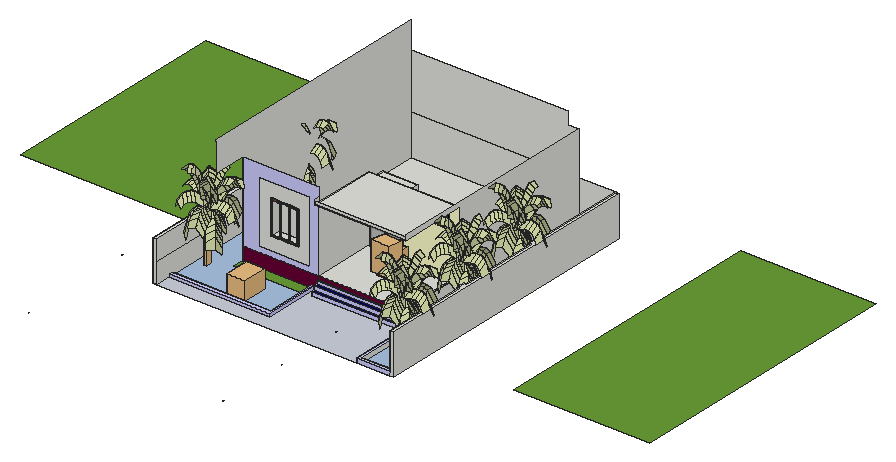
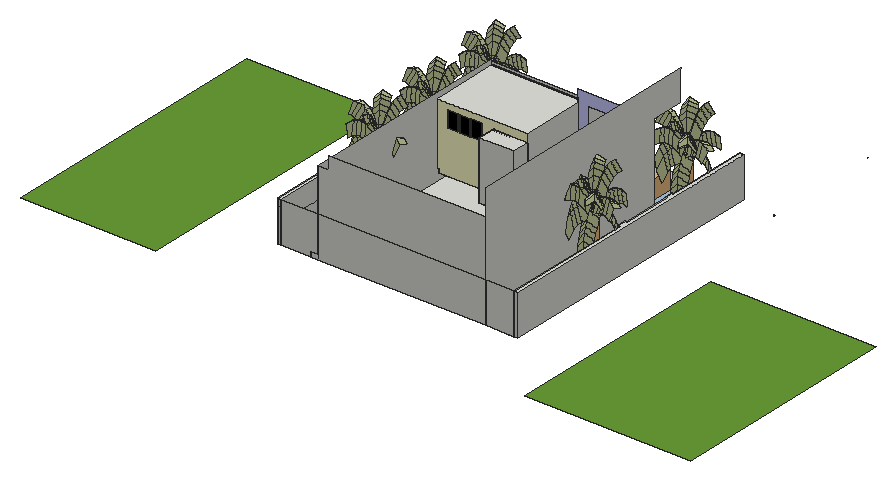
# SketchUp Ruby script. Lengths in inches.
U = 1.inch
M = Sketchup.active_model
def pt(a) = Geom::Point3d.new(a.map { |v| v * U })
def face(e, loops, mat)
  f = e.add_face(loops[0].map { |a| pt(a) })
  loops[1..].each { |l| e.add_face(l.map { |a| pt(a) }).erase! }
  f.material = f.back_material = mat if mat
  f
end
# faces: each face lists its corners as indices into pts; further lists are holes
def faces(e, pts, list, mat = nil) = list.each { |f| face(e, (f[0].is_a?(Array) ? f : [f]).map { |l| l.map { |i| pts[i] } }, mat) }
# xy, xz, yz: faces in a plane at the given z, y or x. An outline is a flat list of corners, or four numbers for a rectangle; further outlines are holes
def ring(l) = l.size == 4 ? [[l[0], l[1]], [l[2], l[1]], [l[2], l[3]], [l[0], l[3]]] : l.each_slice(2).to_a
def flat(e, list, mat, &to3) = list.each { |f| face(e, (f[0].is_a?(Array) ? f : [f]).map { |l| ring(l).map { |u, v| to3.(u, v) } }, mat) }
def xy(e, z, list, mat = nil) = flat(e, list, mat) { |x, y| [x, y, z] }
def xz(e, y, list, mat = nil) = flat(e, list, mat) { |x, z| [x, y, z] }
def yz(e, x, list, mat = nil) = flat(e, list, mat) { |y, z| [x, y, z] }
def lines(e, pts, list) = list.each { |a, b| e.add_line(pt(pts[a]), pt(pts[b])) }
# prism: a flat outline (further loops are holes) pulled along v
def prism(e, loops, v, mat = nil)
  f = face(e, loops, mat); d = Geom::Vector3d.new(v.map { |x| x * U })
  f.pushpull(f.normal.samedirection?(d) ? d.length : -d.length)
end
def box(e, o, s, mat = nil) = prism(e, [[o, [o[0] + s[0], o[1], o[2]], [o[0] + s[0], o[1] + s[1], o[2]], [o[0], o[1] + s[1], o[2]]]], [0, 0, s[2]], mat)
def at(x, y, z, deg = 0) = Geom::Transformation.translation(pt([x, y, z])) * Geom::Transformation.rotation(ORIGIN, Z_AXIS, deg.degrees)
def axes(o, x, y, z) = Geom::Transformation.new([*x, 0, *y, 0, *z, 0, *pt(o).to_a, 1])
def part(name) = M.definitions.add(name)
# library, detail: a bought-in or finely detailed component or shape, given as its bounding box
def library(name, o, s) = part(name).tap { |d| box(d.entities, o, s) }
def detail(e, o, s) = box(e.add_group.entities, o, s)
def put(e, d, t, mat = nil) = e.add_instance(d, t).tap { |i| i.material = mat if mat }
def group(e, t, mat = nil) = e.add_group.tap { |g| g.transformation = t; g.material = mat if mat }.entities
root = M.entities
M.materials.add("Wall-Decor-Art-Painting-YH-W-005-").color = [116, 59, 36]
M.materials.add("Wall-Decor-Art-Painting-YH-W-005- copy").color = [132, 50, 31]
M.materials.add("Wall-Decor-Art-Painting-YH-W-005- copy 2").color = [130, 72, 41]
M.materials.add("Wine2").color = [0, 0, 0]
M.materials["Wine2"].alpha = 0
M.materials.add("[0130_Gainsboro]").color = [39, 45, 50]
M.materials.add("[Color E01]").color = [255, 255, 204]
M.materials.add("[Color I01]").color = [204, 204, 255]
M.materials.add("[Color I08]").color = [0, 0, 102]
M.materials.add("[Color L16]").color = [102, 0, 51]
M.materials.add("[Color M00]").color = [255, 255, 255]
M.materials.add("[Color_002]").color = [198, 198, 198]
M.materials.add("[Color_009]").color = [0, 0, 0]
M.materials.add("[Grass Dark Green]").color = [106, 157, 55]
M.materials.add("[Marble Carrara Floor Tile]").color = [204, 208, 219]
M.materials.add("[Mosaic Hexagonal Tile]").color = [168, 194, 223]
M.materials.add("[Translucent_Resin_Crush_Gray]").color = [184, 184, 184]
M.materials["[Translucent_Resin_Crush_Gray]"].alpha = 0.8
M.materials.add("[Wood Floor Parquet]").color = [145, 89, 39]
M.materials.add("[Wood_Cherry_Original]").color = [152, 86, 42]
M.materials.add("leaf").color = [206, 213, 162]
M.materials.add("top").color = [180, 165, 147]
M.materials.add("Рамы 2").color = [204, 204, 204]
c1 = library("water+(1)",[16,-149.35,-6.82],[116.59,156.63,119.32])
c2 = library("Palm trunk",[157.4375,124.31,0],[15.93,35.48,172.86])
c3 = part("Group\#7")
p = [[164.1,0,77.84],[148.54,0,92.1],[148.54,41.93,119.66],[173.71,41.93,96.59],[148.54,83.86,92.1],[164.1,83.86,77.84],
  [5.38,41.93,118.9],[46.17,41.93,129.83],[46.17,0,102.27],[5.38,0,91.34],[5.38,83.86,91.34],[46.17,83.86,102.27],
  [129.8125,41.93,129.41],[129.8125,0,101.85],[129.8125,83.86,101.85],[109.2,41.93,133.98],[109.2,0,106.42],[109.2,83.86,106.42],
  [88.1,41.93,134.75],[88.1,0,107.19],[88.1,83.86,107.19]]
faces(c3.entities,p,[[0,1,2,3],[3,2,4,5],[6,7,8,9],[10,11,7,6],[12,2,1,13],[14,4,2,12],[15,12,13,16],[17,14,12,15],
  [7,18,19,8],[11,20,18,7],[18,15,16,19],[20,17,15,18]],"leaf")
c4 = part("Coconut palm")
put(c4.entities,c2,at(0,-1.57,0))
put(c4.entities,c3,axes([81.77,133.63,84.54],[0.69255,-0.55067,-0.46599],[0.5,0.83206,-0.24016],[0.51998,-0.06667,0.85157]))
g1 = group(c4.entities,at(162.91,84.37,70.6))
p = [[173.91,67.02,81],[148.54,73.47,103.34],[148.54,106.11,65.23],[164.1,102.16,51.53],[5.38,105.9,64.5],[46.17,108.93,75],
  [46.17,76.29,113.11],[5.38,73.26,102.61],[129.8125,108.8125,74.6],[129.8125,76.17,112.71],[109.2,110.08,78.99],[109.2,77.4375,117.1],
  [164.1,21.59,74.79],[148.54,25.54,88.49],[88.1,110.3,79.73],[88.1,77.65,117.84],[46.17,28.36,98.26],[5.38,25.33,87.76],
  [129.8125,28.24,97.86],[109.2,29.51,102.25],[88.1,29.73,102.99]]
faces(g1,p,[[0,1,2,3],[4,5,6,7],[8,2,1,9],[10,8,9,11],[12,13,1,0],[5,14,15,6],[14,10,11,15],[7,6,16,17],
  [9,1,13,18],[11,9,18,19],[6,15,20,16],[15,11,19,20]],"leaf")
g2 = group(c4.entities,at(165.48,195.56,135.875))
p = [[-108.28,-70.71,-19.53],[-87.32,-105.59,-9.46],[-94.61,-121.11,-48.04],[-115.57,-86.22,-58.11],[-60.61,-153.8125,-57.55],[-53.31,-138.3,-18.96],
  [-98.87,-60.46,-3.65],[-77.9,-95.35,6.42],[-43.9,-128.05,-3.08],[-64.02,-83.84,17.4],[-84.98,-48.95,7.33],[-30.02,-116.54,7.9],
  [-32.71,-60.42,33.34],[-53.67,-25.54,23.27],[1.3,-93.125,23.84],[-18.16,-3.04,27.26],[2.8,-37.93,37.33],[36.81,-70.63,27.83]]
faces(g2,p,[[0,1,2,3],[4,2,1,5],[6,7,1,0],[8,5,1,7],[9,7,6,10],[11,8,7,9],[12,9,10,13],[14,11,9,12],
  [15,16,12,13],[14,12,16,17]],"leaf")
g3 = group(c4.entities,at(142.62,171.34,50.42))
p = [[25.67,-13.71,122.79],[-8.79,-1.2,143.75],[-10.19,32.74,106.83],[24.26,20.24,85.87],[-46.23,10.35,159.48],[-47.64,44.3,122.56],
  [9.41,-59.05,108.76],[-25.04,-46.55,129.72],[-127.77,57.3125,115.67],[-108.71,56.35,124.71],[-107.31,22.41,161.625],[-138.46,23.97,146.85],
  [-66.11,15.49,164.38],[-67.52,49.44,127.46],[-86.76,19.72,165.65],[-88.16,53.67,128.73],[-62.49,-35,145.45],[-123.5625,-22.94,147.59],
  [-142.62,-21.98,138.55],[-82.37,-29.86,150.35],[-103.01,-25.63,151.62]]
faces(g3,p,[[0,1,2,3],[1,4,5,2],[6,7,1,0],[8,9,10,11],[4,12,13,5],[14,10,9,15],[12,14,15,13],[7,16,4,1],
  [11,10,17,18],[16,19,12,4],[20,17,10,14],[19,20,14,12]],"leaf")
g4 = group(c4.entities,at(218.66,104.39,70.49))
p = [[-50.44,173.74,-16.1],[-47.24,168.22,4.03],[-89.48,170.8,30.99],[-95.125,180.54,-4.51],[-127.6875,145.47,10.59],[-130.89,150.99,-9.53],
  [-85.08,160.41,48.83],[-42.84,157.83,21.87],[-123.29,135.08,28.4375],[-79.79,145.86,63.18],[-37.56,143.27,36.22],[-118,120.53,42.79],
  [-74.1,128.98,74.51],[-31.86,126.4,47.55],[-112.31,103.65,54.12],[-62.3,92.16,91.49],[-20.0625,89.58,64.52],[-100.51,66.83,71.09],
  [-50.38,53.24,102.72],[-8.14,50.66,75.76],[-88.59,27.91,82.32]]
faces(g4,p,[[0,1,2,3],[3,2,4,5],[6,2,1,7],[8,4,2,6],[9,6,7,10],[11,8,6,9],[12,9,10,13],[14,11,9,12],
  [15,12,13,16],[17,14,12,15],[18,15,16,19],[20,17,15,18]],"leaf")
g5 = group(c4.entities,at(210.73,128.28,159.9))
p = [[6.68,160.75,-68.99],[43.02,158.53,-41.125],[14.09,136.62,-0.32],[-15.69,143.8,-37.44],[49.16,120.18,15.72],[71.53,137.12,-15.83],
  [-27.22,129.99,-26.4],[2.56,122.8,10.72],[-37.86,112.57,-21],[-8.08,105.38,16.11],[-57.34,75.37,-16.54],[-27.56,68.1875,20.58],
  [-42.45,29.35,13.31],[-72.23,36.53,-23.81],[37.63,106.36,26.76],[27,88.9375,32.16],[-7.375,12.9,29.35],[7.51,51.74,36.62]]
faces(g5,p,[[0,1,2,3],[4,2,1,5],[6,3,2,7],[8,6,7,9],[10,11,12,13],[10,8,9,11],[14,7,2,4],[9,7,14,15],
  [16,12,11,17],[11,9,15,17]],"leaf")
g6 = group(c4.entities,at(98.15,94.13,89.7))
p = [[70.13,63.5,83.51],[57.26,51.26,121.8125],[12.59,51.35,98.97],[25.46,63.59,60.66],[98.15,23.43,72.25],[85.28,11.19,110.5625],
  [42.12,34.09,157.3],[-2.55,34.18,134.45],[70.14,-5.98,146.04],[33.52,23.1,173.14],[-11.15,23.19,150.29],[61.54,-16.97,161.88],
  [23.97,9.59,186.25],[-20.71,9.68,163.41],[51.99,-30.48,175],[13.59,-6.74,194.7],[-31.08,-6.65,171.86],[-41.56,-24.69,175.08],
  [3.11,-24.78,197.92],[41.62,-46.8125,183.45],[31.14,-64.85,186.67]]
faces(g6,p,[[0,1,2,3],[4,5,1,0],[1,6,7,2],[5,8,6,1],[6,9,10,7],[8,11,9,6],[9,12,13,10],[11,14,12,9],
  [12,15,16,13],[17,16,15,18],[14,19,15,12],[18,15,19,20]],"leaf")
g7 = group(c4.entities,at(200.43,222.47,102.78))
p = [[-53.13,-46.15,54.03],[-52.26,-28.65,85.38],[-31.27,-47.33,101.78],[-32.14,-64.84,70.43],[-6,-33.4,86.75],[-6.87,-50.9,55.4],
  [-50.88,-6.91,114.01],[-29.89,-25.6,130.42],[-4.62,-11.66,115.38],[-49.93,5.95,126.57],[-28.94,-12.74,142.97],[-3.67,1.2,127.9375],
  [-48.71,20.77,136.65],[-27.72,2.08,153.05],[-2.45,16.02,138.02],[-47.16,37.54,142.625],[-26.17,18.86,159.03],[-0.9,32.79,144],
  [-23.3125,47.39,161.38],[-45.4,55.14,144.08],[0.86,50.39,145.45]]
faces(g7,p,[[0,1,2,3],[3,2,4,5],[1,6,7,2],[2,7,8,4],[6,9,10,7],[7,10,11,8],[9,12,13,10],[10,13,14,11],
  [12,15,16,13],[13,16,17,14],[18,16,15,19],[20,17,16,18]],"leaf")
g8 = group(c4.entities,at(245.82,148.18,74.1))
p = [[-95.45,43.17,66.56],[-77.22,70.01,93.58],[-59.3125,36.28,126.13],[-77.54,9.45,99.11],[-17.82,13.13,110],[-36.05,-13.7,82.97],
  [-55.78,98.8125,115.8],[-37.87,65.09,148.35],[3.62,41.9375,132.21],[-43.61,113.93,124.1],[-25.69,80.2,156.65],[26.92,133.51,150.95],
  [2.52,110.86,160.76],[-15.39,144.58,128.21],[-0.55,158.36,122.24],[-30.08,129.43,128.85],[-12.17,95.7,161.4],[15.79,57.05,140.52],
  [58.85,101.49,138.66],[44.01,87.71,144.625],[29.32,72.55,145.26]]
faces(g8,p,[[0,1,2,3],[3,2,4,5],[1,6,7,2],[2,7,8,4],[6,9,10,7],[11,12,13,14],[9,15,16,10],[15,13,12,16],
  [7,10,17,8],[18,19,12,11],[10,16,20,17],[16,12,19,20]],"leaf")
g9 = group(c4.entities,at(184.07,231.3125,71.99))
p = [[-52.97,-87.38,70.44],[-75.91,-65.15,98.06],[-38.73,-51.45,128.83],[-15.79,-73.68,101.22],[-10.82,-13.84,110.82],[12.12,-36.07,83.21],
  [-100.5625,-39.55,120.86],[-63.375,-25.85,151.64],[-35.47,11.76,133.625],[-113.51,-25.26,129.46],[-76.32,-11.57,160.23],[-122.54,48.32,155.17],
  [-102.64,20.66,164.86],[-139.82,6.97,134.09],[-151.68,23.45,128.31],[-126.8,-9.65,134.48],[-89.62,4.05,165.25],[-48.42,26.05,142.22],
  [-86.59,74.76,141.07],[-74.73,58.28,146.85],[-61.71,41.66,147.24]]
faces(g9,p,[[0,1,2,3],[3,2,4,5],[1,6,7,2],[2,7,8,4],[6,9,10,7],[11,12,13,14],[9,15,16,10],[7,10,17,8],
  [15,13,12,16],[18,19,12,11],[10,16,20,17],[16,12,19,20]],"leaf")
g10 = group(c4.entities,at(155.33,63.22,90.49))
p = [[56.62,93.99,58],[69.99,76.62,94.09],[26.33,77.04,118.8125],[12.96,94.41,82.72],[-4.99,40.54,104.5],[-18.36,57.91,68.41],
  [85.15,54.53,126.73],[41.49,54.95,151.45],[10.16,18.46,137.14],[93.5,41.24,140.85],[49.84,41.66,165.57],[18.52,5.17,151.26],
  [102.52,25.71,151.94],[58.86,26.125,176.66],[27.53,-10.37,162.35],[111.96,7.84,158.06],[68.3,8.26,182.78],[83.97,-23.96,184],
  [121.19,-11.13,158.78],[36.98,-28.23,168.47],[46.21,-47.21,169.1875]]
faces(g10,p,[[0,1,2,3],[3,2,4,5],[1,6,7,2],[2,7,8,4],[6,9,10,7],[7,10,11,8],[9,12,13,10],[10,13,14,11],
  [12,15,16,13],[17,16,15,18],[13,16,19,14],[20,19,16,17]],"leaf")
g11 = group(c4.entities,at(143.97,131.21,156.06))
p = [[28.02,18.96,27.99],[28.02,5.02,30.3],[22.98,-0.55,-3.35],[22.98,16.04,-6.1],[22.98,22.36,-7.14],[22.98,28.6875,-8.1875],
  [22.98,45.28,-10.9375],[28.02,50.85,22.71],[28.02,36.91,25.02],[28.02,27.9375,26.51],[37.15,27.72,25.18],[51,27.38,23.16],
  [45.96,21.8125,-10.49],[29.41,22.21,-8.08],[16.55,22.52,-6.21],[0,22.92,-3.79],[5.04,28.49,29.86],[18.89,28.16,27.84],
  [29.9,23.86,-8.43],[25,29.125,-8.5625],[30.88,37.53,24.49],[34.36,33.8,24.59],[37.84,30.06,24.6875],[18.08,27.63,-7.28],
  [21.06,35.41,26.3125],[27.89,17.1,-7.01],[34.98,20.46,26.7],[16.0625,20.87,-5.86],[18.19,25.8125,28.33],[25.16,18.34,28.53],
  [20.97,15.61,-5.72],[21.67,22.07,28.43]]
faces(g11,p,[[0,1,2,3,4,5,6,7,8,9],[10,11,12,13,4,14,15,16,17,9],[18,19,20,21,22],[23,24,8,20,19,5],[25,13,18,22,10,26],[17,24,23,14,27,28],[25,26,0,29,30,3],[31,28,27,30,29]],"top")
g12 = group(c4.entities,at(232.25,84.82,92.39))
p = [[-43.76,105.5,48.57],[-18.03,112.66,81.27],[-38.24,79.96,113.53],[-63.96,72.8,80.82],[-25.16,32.38,104.44],[-50.89,25.22,71.74],
  [12.23,118.3125,110.17],[-7.97,85.62,142.42],[5.11,38.03,133.34],[29.42,120.28,122.27],[9.22,87.58,154.52],[48.52,121.17,131.23],
  [28.3125,88.47,163.48],[69.25,120.47,135.17],[49.04,87.77,167.43],[22.3,40,145.4375],[84.11,84.01,165.18],[90.19,118.22,133.83],
  [41.39,40.89,154.4],[62.12,40.1875,158.34],[83.07,37.94,157]]
faces(g12,p,[[0,1,2,3],[3,2,4,5],[1,6,7,2],[2,7,8,4],[6,9,10,7],[9,11,12,10],[11,13,14,12],[7,10,15,8],
  [16,14,13,17],[10,12,18,15],[12,14,19,18],[20,19,14,16]],"leaf")
g13 = group(c4.entities,at(137.93,152.93,50.82))
p = [[30.35,4.7,122.39],[5.92,-23.64,141.95],[-27.65,-7.16,108.51],[-3.22,21.19,88.95],[63.93,-27.07,102.88],[39.49,-55.42,122.4375],
  [-19.2,-54.54,156],[-52.77,-38.05,122.55],[-98.3,-104.66,111.23],[-88.98,-88.73,121.47],[-55.4,-105.22,154.92],[-70.46,-130.95,138.37],
  [-44.1875,-88.11,160.125],[-77.76,-71.62,126.68],[14.375,-86.32,136.48],[-31.84,-70.99,159.9375],[-65.41,-54.5,126.49],[-21.83,-137,135.4],
  [-31.15,-152.93,125.16],[-10.61,-119.89,140.61],[1.73,-102.76,140.42]]
faces(g13,p,[[0,1,2,3],[4,5,1,0],[1,6,7,2],[8,9,10,11],[12,10,9,13],[5,14,6,1],[6,15,16,7],[11,10,17,18],
  [15,12,13,16],[19,17,10,12],[14,20,15,6],[20,19,12,15]],"leaf")
put(c4.entities,c3,axes([95.25,164,66.31],[0.22415,-0.97195,-0.07116],[0.94191,0.2348,-0.24016],[0.25014,-0.0132,0.96812]))
c5 = part("coconut (1)")
xy(c5.entities,0,[[0,37.8,1,38.8,1,37.8]])
put(c5.entities,c4,at(217.64,826.21,0))
c6 = part("Group\#69")
xy(c6.entities,0,[[0.79,0.6875,0.23,0.83,0,1.16,0.23,1.5,0.79,1.63,1.34,1.5,1.57,1.16,1.34,0.83]],"[Color_002]")
xy(c6.entities,5.31,[[0.69,0,0.69,0.71,0.79,0.6875,0.88,0.71,0.88,0]],"[Color_002]")
xy(c6.entities,6.35,[[0.69,0,0.88,0,0.88,0.71,0.79,0.6875,0.69,0.71]],"[Color_002]")
xy(c6.entities,9.4,[[0.69,0,0.69,0.71,0.79,0.6875,0.88,0.71,0.88,0]],"[Color_002]")
xy(c6.entities,10.44,[[0.69,0,0.88,0,0.88,0.71,0.79,0.6875,0.69,0.71]],"[Color_002]")
xy(c6.entities,15.75,[[0.79,0.6875,1.34,0.83,1.57,1.16,1.34,1.5,0.79,1.63,0.23,1.5,0,1.16,0.23,0.83]],"[Color_002]")
xz(c6.entities,0,[[0.69,5.31,0.88,6.35],[0.69,9.4,0.88,10.44]],"[Color_002]")
yz(c6.entities,0.69,[[0,5.31,0.71,6.35],[0,9.4,0.71,10.44]],"[Color_002]")
yz(c6.entities,0.88,[[0,5.31,0.71,6.35],[0,9.4,0.71,10.44]],"[Color_002]")
p = [[0.23,0.83,0],[0.79,0.6875,0],[0.79,0.6875,5.31],[0.79,0.6875,6.35],[0.79,0.6875,9.4],[0.79,0.6875,10.44],
  [0.79,0.6875,15.75],[0.23,0.83,15.75],[1.34,0.83,0],[1.34,0.83,15.75],[0,1.16,0],[0,1.16,15.75],
  [1.57,1.16,0],[1.57,1.16,15.75],[0.23,1.5,0],[0.23,1.5,15.75],[1.34,1.5,0],[1.34,1.5,15.75],
  [0.79,1.63,0],[0.79,1.63,15.75]]
faces(c6.entities,p,[[0,1,2,3,4,5,6,7],[1,8,9,6,5,4,3,2],[10,0,7,11],[8,12,13,9],[14,10,11,15],[12,16,17,13],[18,14,15,19],[16,18,19,17]],"[Color_002]")
c7 = part("door 2")
g14 = group(c7.entities,at(-1.57,-0.59,0))
xy(g14,0,[[0,0,2.76,0.59],[31.89,0,34.65,0.59],[0,3.74,2.76,4.33],[31.89,3.74,34.65,4.33]])
xy(g14,1.97,[[4.72,1.18,29.92,2.17],[4.72,2.17,29.92,3.15]],"Рамы 2")
xy(g14,79.53,[[4.72,1.18,29.92,2.17],[4.72,2.17,29.92,3.15]],"Рамы 2")
xy(g14,81.5,[[2.76,0,31.89,1.18],[2.76,3.15,31.89,4.33]],"[Wood_Cherry_Original]")
xy(g14,84.25,[[0,0,34.65,0.59],[0,3.74,34.65,4.33]],"[Wood_Cherry_Original]")
xz(g14,0,[[0,0,2.76,0,2.76,81.5,31.89,81.5,31.89,0,34.65,0,34.65,84.25,0,84.25]],"[Wood_Cherry_Original]")
xz(g14,1.18,[[[2.76,0,31.89,81.5],[4.72,1.97,29.92,79.53]]],"Рамы 2")
xz(g14,2.17,[[4.72,1.97,29.92,79.53]],"[Translucent_Resin_Crush_Gray]")
xz(g14,3.15,[[[2.76,0,31.89,81.5],[4.72,1.97,29.92,79.53]]],"Рамы 2")
xz(g14,4.33,[[0,0,0,84.25,34.65,84.25,34.65,0,31.89,0,31.89,81.5,2.76,81.5,2.76,0]],"[Wood_Cherry_Original]")
yz(g14,0,[[0,0,0.59,84.25],[3.74,0,4.33,84.25]],"[Wood_Cherry_Original]")
yz(g14,2.76,[[0,0,1.18,81.5],[3.15,0,4.33,81.5]],"[Wood_Cherry_Original]")
yz(g14,4.72,[[1.18,1.97,2.17,79.53],[2.17,1.97,3.15,79.53]],"Рамы 2")
yz(g14,29.92,[[1.18,1.97,2.17,79.53],[2.17,1.97,3.15,79.53]],"Рамы 2")
yz(g14,31.89,[[0,0,1.18,81.5],[3.15,0,4.33,81.5]],"[Wood_Cherry_Original]")
yz(g14,34.65,[[3.74,0,4.33,84.25]])
yz(g14,34.65,[[0,0,0.59,84.25]],"[Wood_Cherry_Original]")
put(c7.entities,c6,at(27.96,2.56,33.02))
put(c7.entities,c6,axes([27.96,0.59,33.02],[1,0,0],[0,-1,0],[0,0,1]))
c8 = library("314-401",[-12.02,-0.78,-0.35],[24.04,20.75,31.48])
c9 = library("Group1\#1",[-12.04,-13.74,-0.03],[39.22,27.79,53.13])
c10 = part("rttfff")
g15 = group(c10.entities,at(53.02,40.46,1.02))
xy(g15,0,[[0,-1.21,14.3,0]],"[Color_009]")
xy(g15,38.86,[[0,-1.21,14.3,0]],"[Color_009]")
xz(g15,-1.21,[[0,0,14.3,38.86]],"Wall-Decor-Art-Painting-YH-W-005-")
xz(g15,0,[[0,0,14.3,38.86]],"[Color_009]")
yz(g15,0,[[-1.21,0,0,38.86]],"[Color_009]")
yz(g15,14.3,[[-1.21,0,0,38.86]],"[Color_009]")
g16 = group(c10.entities,at(85.5,40.46,1.02))
xy(g16,0,[[0,-1.21,14.3,0]],"[Color_009]")
xy(g16,38.86,[[0,-1.21,14.3,0]],"[Color_009]")
xz(g16,-1.21,[[0,0,14.3,38.86]],"Wall-Decor-Art-Painting-YH-W-005- copy")
xz(g16,0,[[0,0,14.3,38.86]],"[Color_009]")
yz(g16,0,[[-1.21,0,0,38.86]],"[Color_009]")
yz(g16,14.3,[[-1.21,0,0,38.86]],"[Color_009]")
g17 = group(c10.entities,at(69.26,40.46,1.02))
xy(g17,0,[[0,-1.21,14.3,0]],"[Color_009]")
xy(g17,38.86,[[0,-1.21,14.3,0]],"[Color_009]")
xz(g17,-1.21,[[0,0,14.3,38.86]],"Wall-Decor-Art-Painting-YH-W-005- copy 2")
xz(g17,0,[[0,0,14.3,38.86]],"[Color_009]")
yz(g17,0,[[-1.21,0,0,38.86]],"[Color_009]")
yz(g17,14.3,[[-1.21,0,0,38.86]],"[Color_009]")
xy(root,-52.93,[[3367.8,1060.11,4222.3,2841.86],[0,1380.97,1044.44,2841.86]],"[Grass Dark Green]")
xy(root,0,[[1372.11,712.05,1396.4375,712.05,1396.4375,806.17,2030.3125,806.17,2030.3125,1158.61,2058.38,1158.61,2058.38,1100.29,2631.21,1100.29,2631.21,1158.61,2657.4,1158.61,2657.4,712.05,2865.28,712.05,2865.28,725.25,2676.2,725.25,2676.2,2487.49,1576.31,2487.49,1576.31,1158.61,2016.25,1158.61,2016.25,832.36,1396.4375,832.36,1396.4375,2487.49,1372.11,2487.49],[2865.28,712.05,2887.11,2487.49]])
xy(root,0,[[1576.31,1091.78,2016.25,1158.61]],"[Grass Dark Green]")
xy(root,0,[[1396.4375,712.05,2657.4,712.05,2657.4,1158.61,2631.21,1158.61,2631.21,1100.29,2058.38,1100.29,2058.38,1158.61,2030.3125,1158.61,2030.3125,806.17,1396.4375,806.17]],"[Marble Carrara Floor Tile]")
xy(root,0,[[2676.2,725.25,2865.28,2487.49],[1396.4375,832.36,2016.25,832.36,2016.25,1091.78,1576.31,1091.78,1576.31,2487.49,1396.4375,2487.49]],"[Mosaic Hexagonal Tile]")
xy(root,17.0625,[[1396.4375,806.17,2030.3125,806.17,2030.3125,1158.61,2016.25,1158.61,2016.25,832.36,1396.4375,832.36]],"[Color I01]")
xy(root,21.125,[[2058.38,1100.29,2631.21,1119.42]],"[Color I08]")
xy(root,30.9375,[[2657.4,712.05,2865.28,712.05,2865.28,725.25,2676.2,725.25,2676.2,2487.49,2631.21,2487.49,2631.21,1158.61,2657.4,1158.61]],"[Color I01]")
xy(root,44.21,[[2058.38,1119.42,2631.21,1143.54]],"[Color I08]")
xy(root,61.74,[[2058.38,1143.54,2631.21,1158.61]],"[Color I08]")
xy(root,86.0625,[[2058.38,1158.61,2619.08,1158.61,2619.08,1553.21,2274.25,1553.21,2274.25,1664.71,2058.38,1664.71]])
xy(root,108.125,[[2619.08,1158.61,2631.21,1553.21]])
xy(root,128.25,[[1396.4375,1233.8125,1406,1282.32],[2852.9,1253.21,2865.28,1309.98],[1396.4375,1596.58,1408.9375,1656.72],[2848.65,1819.47,2865.28,1898.73]])
xy(root,206.05,[[1758.91,1158.61,1930.16,1219.92]])
xy(root,206.05,[[1758.91,1158.03,1815.07,1158.27],[1815.07,1158.03,1871.22,1158.27],[1871.22,1158.03,1927.38,1158.27],[1758.91,1158.27,1815.07,1158.61],[1815.07,1158.27,1871.22,1158.61],
  [1871.22,1158.27,1927.38,1158.61]],"[0130_Gainsboro]")
xy(root,206.61,[[1759.31,1157.93,1814.67,1158.03],[1815.46,1157.93,1870.83,1158.03],[1871.62,1157.93,1926.98,1158.03]],"[0130_Gainsboro]")
xy(root,211.47,[[1762.76,1157.93,1811.22,1158.12],[1818.92,1157.93,1867.375,1158.12],[1875.07,1157.93,1923.53,1158.12],[1762.76,1158.12,1811.22,1158.27],[1818.92,1158.12,1867.375,1158.27],
  [1875.07,1158.12,1923.53,1158.27],[1762.76,1158.27,1811.22,1158.42],[1818.92,1158.27,1867.375,1158.42],[1875.07,1158.27,1923.53,1158.42],[1762.76,1158.42,1811.22,1158.61],
  [1818.92,1158.42,1867.375,1158.61],[1875.07,1158.42,1923.53,1158.61]],"[0130_Gainsboro]")
xy(root,212.55,[[1763.53,1158.12,1810.45,1158.27],[1819.68,1158.12,1866.61,1158.27],[1875.84,1158.12,1922.76,1158.27],[1763.53,1158.27,1810.45,1158.42],[1819.68,1158.27,1866.61,1158.42],
  [1875.84,1158.27,1922.76,1158.42]],"[0130_Gainsboro]")
xy(root,256.5,[[1372.11,712.05,1396.4375,712.05,1396.4375,1233.8125,1406,1233.8125,1406,1282.32,1396.4375,1282.32,1396.4375,1596.58,1408.9375,1596.58,1408.9375,1656.72,1396.4375,1656.72,1396.4375,2487.49,1372.11,2487.49],[2865.28,712.05,2887.11,712.05,2887.11,2487.49,2865.28,2487.49,2865.28,1898.73,2848.65,1898.73,2848.65,1819.47,2865.28,1819.47,2865.28,1309.98,2852.9,1309.98,2852.9,1253.21,2865.28,1253.21]])
xy(root,411.36,[[1763.53,1158.12,1810.45,1158.27],[1819.68,1158.12,1866.61,1158.27],[1875.84,1158.12,1922.76,1158.27],[1763.53,1158.27,1810.45,1158.42],[1819.68,1158.27,1866.61,1158.42],
  [1875.84,1158.27,1922.76,1158.42]],"[0130_Gainsboro]")
xy(root,412.44,[[1762.76,1157.93,1811.22,1158.12],[1818.92,1157.93,1867.375,1158.12],[1875.07,1157.93,1923.53,1158.12],[1762.76,1158.12,1811.22,1158.27],[1818.92,1158.12,1867.375,1158.27],
  [1875.07,1158.12,1923.53,1158.27],[1762.76,1158.27,1811.22,1158.42],[1818.92,1158.27,1867.375,1158.42],[1875.07,1158.27,1923.53,1158.42],[1762.76,1158.42,1811.22,1158.61],
  [1818.92,1158.42,1867.375,1158.61],[1875.07,1158.42,1923.53,1158.61]],"[0130_Gainsboro]")
xy(root,417.31,[[1759.31,1157.93,1814.67,1158.03],[1815.46,1157.93,1870.83,1158.03],[1871.62,1157.93,1926.98,1158.03]],"[0130_Gainsboro]")
xy(root,417.86,[[1758.91,1158.61,1930.16,1219.92]])
xy(root,417.86,[[1758.91,1158.03,1815.07,1158.27],[1815.07,1158.03,1871.22,1158.27],[1871.22,1158.03,1927.38,1158.27],[1758.91,1158.27,1815.07,1158.61],[1815.07,1158.27,1871.22,1158.61],
  [1871.22,1158.27,1927.38,1158.61]],"[0130_Gainsboro]")
xy(root,452.6875,[[2058.38,1553.21,2274.25,1664.71]])
xy(root,499.87,[[2058.38,1124.92,2631.21,1553.21]])
xy(root,504.41,[[2058.38,1123.42,2631.21,1124.92]])
xz(root,712.05,[[1372.11,0,1396.4375,256.5],[2865.28,0,2887.11,256.5]])
xz(root,712.05,[[2657.4,0,2865.28,30.9375]],"[Color I01]")
xz(root,725.25,[[2676.2,0,2865.28,30.9375]])
xz(root,806.17,[[1396.4375,0,2030.3125,17.0625]],"[Color I01]")
xz(root,832.36,[[1396.4375,0,2016.25,17.0625]])
xz(root,1100.29,[[2058.38,0,2631.21,21.125]],"[Color I01]")
xz(root,1119.42,[[2058.38,21.125,2631.21,44.21]],"[Color I01]")
xz(root,1123.42,[[2058.38,504.41,2631.21,523.46]])
xz(root,1124.92,[[2058.38,499.87,2631.21,504.41]])
xz(root,1143.54,[[2058.38,44.21,2631.21,61.74]],"[Color I01]")
xz(root,1157.93,[[[1759.31,206.61,1814.67,417.31],[1762.76,211.47,1811.22,412.44]],[[1815.46,206.61,1870.83,417.31],[1818.92,211.47,1867.375,412.44]],[[1871.62,206.61,1926.98,417.31],[1875.07,211.47,1923.53,412.44]]],"[Wood Floor Parquet]")
xz(root,1158.03,[[[1758.91,206.05,1815.07,417.86],[1759.31,206.61,1814.67,417.31]],[[1815.07,206.05,1871.22,417.86],[1815.46,206.61,1870.83,417.31]],[[1871.22,206.05,1927.38,417.86],[1871.62,206.61,1926.98,417.31]]],"[0130_Gainsboro]")
xz(root,1158.12,[[[1762.76,211.47,1811.22,412.44],[1763.53,212.55,1810.45,411.36]],[[1818.92,211.47,1867.375,412.44],[1819.68,212.55,1866.61,411.36]],[[1875.07,211.47,1923.53,412.44],[1875.84,212.55,1922.76,411.36]]],"[0130_Gainsboro]")
xz(root,1158.27,[[1763.53,212.55,1810.45,411.36],[1819.68,212.55,1866.61,411.36],[1875.84,212.55,1922.76,411.36]],"Wine2")
xz(root,1158.27,[[[1758.91,206.05,1815.07,417.86],[1762.76,211.47,1811.22,412.44]],[[1815.07,206.05,1871.22,417.86],[1818.92,211.47,1867.375,412.44]],[[1871.22,206.05,1927.38,417.86],[1875.07,211.47,1923.53,412.44]],[[1762.76,211.47,1811.22,412.44],[1763.53,212.55,1810.45,411.36]],[[1818.92,211.47,1867.375,412.44],[1819.68,212.55,1866.61,411.36]],
  [[1875.07,211.47,1923.53,412.44],[1875.84,212.55,1922.76,411.36]]],"[0130_Gainsboro]")
xz(root,1158.42,[[[1762.76,211.47,1811.22,412.44],[1763.53,212.55,1810.45,411.36]],[[1818.92,211.47,1867.375,412.44],[1819.68,212.55,1866.61,411.36]],[[1875.07,211.47,1923.53,412.44],[1875.84,212.55,1922.76,411.36]]],"[0130_Gainsboro]")
xz(root,1158.61,[[2631.21,0,2657.4,30.9375],[[1685.6,122.14,1996.97,509.14],[1758.91,206.05,1930.16,417.86]]])
xz(root,1158.61,[[[1758.91,206.05,1815.07,417.86],[1762.76,211.47,1811.22,412.44]],[[1815.07,206.05,1871.22,417.86],[1818.92,211.47,1867.375,412.44]],[[1871.22,206.05,1927.38,417.86],[1875.07,211.47,1923.53,412.44]]],"[0130_Gainsboro]")
xz(root,1158.61,[[[1576.31,86.0625,2058.38,584.23],[1685.6,122.14,1996.97,509.14]]],"[Color I01]")
xz(root,1158.61,[[1576.31,0,2016.25,0,2016.25,17.0625,2030.3125,17.0625,2030.3125,0,2058.38,0,2058.38,86.0625,1576.31,86.0625],[2058.38,61.74,2631.21,61.74,2631.21,108.125,2619.08,108.125,2619.08,86.0625,2058.38,86.0625]],"[Color L16]")
xz(root,1219.92,[[1758.91,206.05,1930.16,417.86]])
xz(root,1233.8125,[[1396.4375,128.25,1406,256.5]],"[Color M00]")
xz(root,1253.21,[[2852.9,128.25,2865.28,256.5]],"[Color M00]")
xz(root,1282.32,[[1396.4375,128.25,1406,256.5]])
xz(root,1309.98,[[2852.9,128.25,2865.28,256.5]])
xz(root,1553.21,[[2274.25,86.0625,2619.08,86.0625,2619.08,108.125,2631.21,108.125,2631.21,499.87,2058.38,499.87,2058.38,452.6875,2274.25,452.6875]],"[Color E01]")
xz(root,1596.58,[[1396.4375,128.25,1408.9375,256.5]],"[Color M00]")
xz(root,1656.72,[[1396.4375,128.25,1408.9375,256.5]])
xz(root,1664.71,[[2058.38,86.0625,2274.25,452.6875]])
xz(root,1819.47,[[2848.65,128.25,2865.28,256.5]],"[Color M00]")
xz(root,1898.73,[[2848.65,128.25,2865.28,256.5]])
xz(root,2487.49,[[1372.11,0,1396.4375,256.5],[1396.4375,0,1576.31,256.5],[1576.31,0,2631.21,256.5],[2631.21,0,2676.2,30.9375],[2676.2,0,2676.2,30.9375,2631.21,30.9375,2631.21,256.5,2865.28,256.5,2865.28,0],
  [2865.28,0,2887.11,216.4375],[2865.28,216.4375,2887.11,256.5],[1576.31,256.5,1576.31,609.375,2562.14,609.375,2562.14,530.44,2631.21,530.44,2631.21,256.5]])
yz(root,1372.11,[[712.05,0,2487.49,256.5]])
yz(root,1396.4375,[[712.05,0,806.17,0,806.17,17.0625,832.36,17.0625,832.36,0,2487.49,0,2487.49,128.25,712.05,128.25],[712.05,128.25,1233.8125,256.5],[1282.32,128.25,1596.58,256.5],[1656.72,128.25,2487.49,256.5]])
yz(root,1406,[[1233.8125,128.25,1282.32,256.5]],"[Color M00]")
yz(root,1408.9375,[[1596.58,128.25,1656.72,256.5]],"[Color M00]")
yz(root,1576.31,[[1158.61,0,1158.61,584.23,956.92,584.23,956.92,769.62,947.29,769.62,947.29,774.9375,2487.49,774.9375,2487.49,0]])
yz(root,1758.91,[[1158.61,206.05,1219.92,417.86]])
yz(root,1758.91,[[1158.03,206.05,1158.27,417.86],[1158.27,206.05,1158.61,417.86]],"[0130_Gainsboro]")
yz(root,1759.31,[[1157.93,206.61,1158.03,417.31]],"[0130_Gainsboro]")
yz(root,1762.76,[[1157.93,211.47,1158.12,412.44],[1158.12,211.47,1158.27,412.44],[1158.27,211.47,1158.42,412.44],[1158.42,211.47,1158.61,412.44]],"[0130_Gainsboro]")
yz(root,1763.53,[[1158.12,212.55,1158.27,411.36],[1158.27,212.55,1158.42,411.36]],"[0130_Gainsboro]")
yz(root,1810.45,[[1158.12,212.55,1158.27,411.36],[1158.27,212.55,1158.42,411.36]],"[0130_Gainsboro]")
yz(root,1811.22,[[1157.93,211.47,1158.12,412.44],[1158.12,211.47,1158.27,412.44],[1158.27,211.47,1158.42,412.44],[1158.42,211.47,1158.61,412.44]],"[0130_Gainsboro]")
yz(root,1814.67,[[1157.93,206.61,1158.03,417.31]],"[0130_Gainsboro]")
yz(root,1815.07,[[1158.03,206.05,1158.27,417.86],[1158.27,206.05,1158.61,417.86]],"[0130_Gainsboro]")
yz(root,1815.46,[[1157.93,206.61,1158.03,417.31]],"[0130_Gainsboro]")
yz(root,1818.92,[[1157.93,211.47,1158.12,412.44],[1158.12,211.47,1158.27,412.44],[1158.27,211.47,1158.42,412.44],[1158.42,211.47,1158.61,412.44]],"[0130_Gainsboro]")
yz(root,1819.68,[[1158.12,212.55,1158.27,411.36],[1158.27,212.55,1158.42,411.36]],"[0130_Gainsboro]")
yz(root,1866.61,[[1158.12,212.55,1158.27,411.36],[1158.27,212.55,1158.42,411.36]],"[0130_Gainsboro]")
yz(root,1867.375,[[1157.93,211.47,1158.12,412.44],[1158.12,211.47,1158.27,412.44],[1158.27,211.47,1158.42,412.44],[1158.42,211.47,1158.61,412.44]],"[0130_Gainsboro]")
yz(root,1870.83,[[1157.93,206.61,1158.03,417.31]],"[0130_Gainsboro]")
yz(root,1871.22,[[1158.03,206.05,1158.27,417.86],[1158.27,206.05,1158.61,417.86]],"[0130_Gainsboro]")
yz(root,1871.62,[[1157.93,206.61,1158.03,417.31]],"[0130_Gainsboro]")
yz(root,1875.07,[[1157.93,211.47,1158.12,412.44],[1158.12,211.47,1158.27,412.44],[1158.27,211.47,1158.42,412.44],[1158.42,211.47,1158.61,412.44]],"[0130_Gainsboro]")
yz(root,1875.84,[[1158.12,212.55,1158.27,411.36],[1158.27,212.55,1158.42,411.36]],"[0130_Gainsboro]")
yz(root,1922.76,[[1158.12,212.55,1158.27,411.36],[1158.27,212.55,1158.42,411.36]],"[0130_Gainsboro]")
yz(root,1923.53,[[1157.93,211.47,1158.12,412.44],[1158.12,211.47,1158.27,412.44],[1158.27,211.47,1158.42,412.44],[1158.42,211.47,1158.61,412.44]],"[0130_Gainsboro]")
yz(root,1926.98,[[1157.93,206.61,1158.03,417.31]],"[0130_Gainsboro]")
yz(root,1927.38,[[1158.03,206.05,1158.27,417.86],[1158.27,206.05,1158.61,417.86]],"[0130_Gainsboro]")
yz(root,1930.16,[[1158.61,206.05,1219.92,417.86]])
yz(root,2016.25,[[832.36,0,1158.61,17.0625]],"[Color I01]")
yz(root,2030.3125,[[806.17,0,1158.61,17.0625]],"[Color I01]")
yz(root,2058.38,[[1100.29,0,1100.29,21.125,1119.42,21.125,1119.42,30.9375,1158.61,30.9375,1158.61,0],[1119.42,30.9375,1119.42,44.21,1143.54,44.21,1143.54,49.84,1158.61,49.84,1158.61,30.9375],[1143.54,49.84,1158.61,61.74],[1158.61,86.0625,1664.71,86.0625,1664.71,452.6875,1553.21,452.6875,1553.21,499.87,1158.61,499.87],[1124.92,499.87,1124.92,504.41,1123.42,504.41,1123.42,523.46,1124.92,523.46,1124.92,530.44,1158.61,530.44,1158.61,499.87]])
yz(root,2274.25,[[1553.21,86.0625,1664.71,452.6875]])
yz(root,2619.08,[[1158.61,86.0625,1553.21,108.125]])
yz(root,2631.21,[[1100.29,0,1158.61,0,1158.61,30.9375,1119.42,30.9375,1119.42,21.125,1100.29,21.125],[1119.42,30.9375,2487.49,30.9375,2487.49,530.44,1124.92,530.44,1124.92,523.46,1123.42,523.46,1123.42,504.41,1124.92,504.41,1124.92,499.87,1553.21,499.87,1553.21,108.125,1158.61,108.125,1158.61,61.74,1143.54,61.74,1143.54,44.21,1119.42,44.21]])
yz(root,2657.4,[[712.05,0,1158.61,30.9375]],"[Color I01]")
yz(root,2676.2,[[725.25,0,2487.49,30.9375]])
yz(root,2848.65,[[1819.47,128.25,1898.73,256.5]],"[Color M00]")
yz(root,2852.9,[[1253.21,128.25,1309.98,256.5]],"[Color M00]")
yz(root,2865.28,[[725.25,0,725.25,30.9375,712.05,30.9375,712.05,128.25,2487.49,128.25,2487.49,0],[712.05,128.25,1253.21,256.5],[1309.98,128.25,1819.47,256.5],[1898.73,128.25,2487.49,256.5]])
yz(root,2887.11,[[712.05,0,2487.49,256.5]])
put(root,c1,at(2672.42,1669.27,-0.1875))
put(root,c1,at(2672.42,1180.77,-0.1875))
put(root,c1,at(1702.73,1004.77,0))
put(root,c5,axes([2381.78,425.77,0],[1,0,0],[0,1,0],[0,0,2]))
put(root,c5,axes([2381.78,852.89,0],[1,0,0],[0,1,0],[0,0,2]))
put(root,c5,axes([2381.78,-37.8,0],[1,0,0],[0,1,0],[0,0,2]))
put(root,c5,axes([1117.89,747.92,34.125],[1,0,0],[0,1,0],[0,0,2]))
put(root,c5,axes([1117.89,12.85,34.125],[1,0,0],[0,1,0],[0,0,2]))
put(root,c7,axes([2270.67,1546.67,86.0625],[-3.19813,0,0],[0,4.62536,0],[0,0,4.32765]))
put(root,c7,axes([2062.14,1551.96,86.0625],[3.39,0,0],[0,0.29925,0],[0,0,4.32765]))
put(root,c8,axes([2368.7,1290.22,128.8],[3.6556,0,0],[0,6.2624,0],[0,0,4.1553]))
put(root,c9,axes([2373.92,1317.9,152.28],[-0.45397,-2.1301,0],[4.17891,-0.2314,0],[0,0,3.41268]))
put(root,c10,axes([2109.03,1314.36,355.68],[4.52037,0,0],[0,5.90402,0],[0,0,2.59038]))
